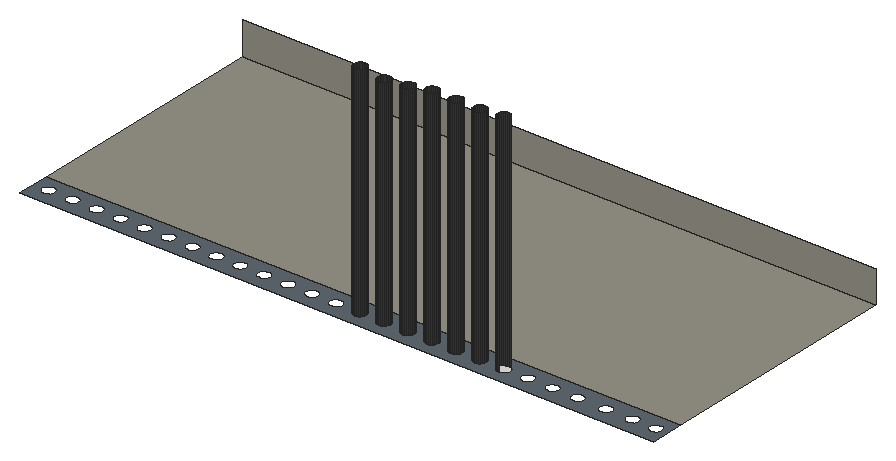
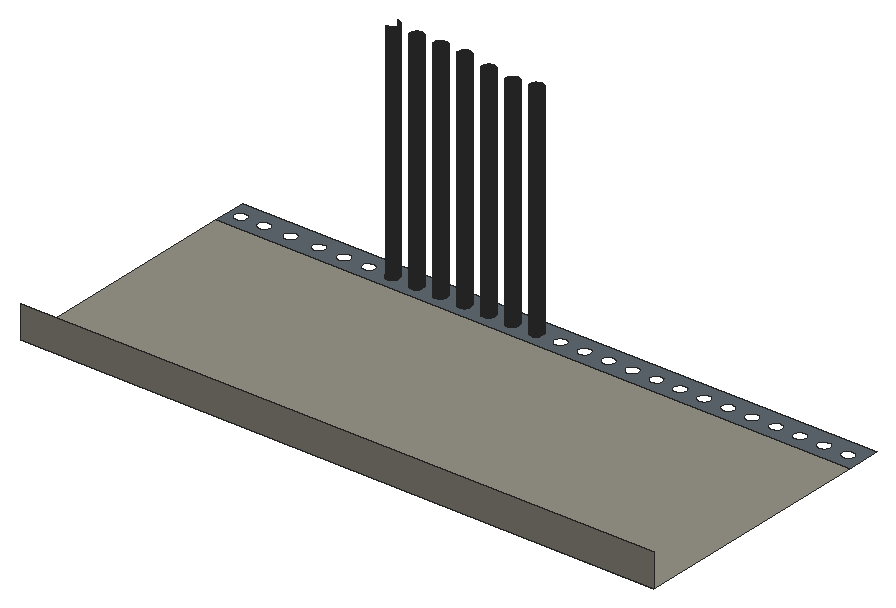
# SketchUp Ruby script. Lengths in inches.
U = 1.inch
M = Sketchup.active_model
def pt(a) = Geom::Point3d.new(a.map { |v| v * U })
def face(e, loops, mat)
  f = e.add_face(loops[0].map { |a| pt(a) })
  loops[1..].each { |l| e.add_face(l.map { |a| pt(a) }).erase! }
  f.material = f.back_material = mat if mat
  f
end
# faces: each face lists its corners as indices into pts; further lists are holes
def faces(e, pts, list, mat = nil) = list.each { |f| face(e, (f[0].is_a?(Array) ? f : [f]).map { |l| l.map { |i| pts[i] } }, mat) }
# xy, xz, yz: faces in a plane at the given z, y or x. An outline is a flat list of corners, or four numbers for a rectangle; further outlines are holes
def ring(l) = l.size == 4 ? [[l[0], l[1]], [l[2], l[1]], [l[2], l[3]], [l[0], l[3]]] : l.each_slice(2).to_a
def flat(e, list, mat, &to3) = list.each { |f| face(e, (f[0].is_a?(Array) ? f : [f]).map { |l| ring(l).map { |u, v| to3.(u, v) } }, mat) }
def xy(e, z, list, mat = nil) = flat(e, list, mat) { |x, y| [x, y, z] }
def xz(e, y, list, mat = nil) = flat(e, list, mat) { |x, z| [x, y, z] }
def yz(e, x, list, mat = nil) = flat(e, list, mat) { |y, z| [x, y, z] }
def lines(e, pts, list) = list.each { |a, b| e.add_line(pt(pts[a]), pt(pts[b])) }
# prism: a flat outline (further loops are holes) pulled along v
def prism(e, loops, v, mat = nil)
  f = face(e, loops, mat); d = Geom::Vector3d.new(v.map { |x| x * U })
  f.pushpull(f.normal.samedirection?(d) ? d.length : -d.length)
end
def box(e, o, s, mat = nil) = prism(e, [[o, [o[0] + s[0], o[1], o[2]], [o[0] + s[0], o[1] + s[1], o[2]], [o[0], o[1] + s[1], o[2]]]], [0, 0, s[2]], mat)
def at(x, y, z, deg = 0) = Geom::Transformation.translation(pt([x, y, z])) * Geom::Transformation.rotation(ORIGIN, Z_AXIS, deg.degrees)
def axes(o, x, y, z) = Geom::Transformation.new([*x, 0, *y, 0, *z, 0, *pt(o).to_a, 1])
def part(name) = M.definitions.add(name)
# library, detail: a bought-in or finely detailed component or shape, given as its bounding box
def library(name, o, s) = part(name).tap { |d| box(d.entities, o, s) }
def detail(e, o, s) = box(e.add_group.entities, o, s)
def put(e, d, t, mat = nil) = e.add_instance(d, t).tap { |i| i.material = mat if mat }
def group(e, t, mat = nil) = e.add_group.tap { |g| g.transformation = t; g.material = mat if mat }.entities
root = M.entities
M.materials.add("[Color M07]").color = [58, 58, 58]
M.materials.add("[Formica Graystone]").color = [149, 146, 135]
M.materials.add("[Formica Speckled Grey]").color = [94, 105, 111]
xy(root,557.29,[[258.98,117.55,258.8125,117.57,258.66,117.63,258.53,117.73,258.43,117.86,258.37,118.01,258.35,118.17,258.37,118.33,258.43,118.48,258.53,118.61,258.66,118.71,258.8125,118.77,258.98,118.8,259.14,118.77,259.29,118.71,259.42,118.61,259.52,118.48,259.58,118.33,259.6,118.17,259.58,118.01,259.52,117.86,259.42,117.73,259.29,117.63,259.14,117.57],[261.35,117.55,261.1875,117.57,261.04,117.63,260.91,117.73,260.81,117.86,260.75,118.01,260.73,118.17,260.75,118.33,260.81,118.48,260.91,118.61,261.04,118.71,261.1875,118.77,261.35,118.8,261.51,118.77,261.66,118.71,261.79,118.61,261.89,118.48,261.95,118.33,261.98,118.17,261.95,118.01,261.89,117.86,261.79,117.73,261.66,117.63,261.51,117.57],[263.73,117.55,263.5625,117.57,263.41,117.63,263.28,117.73,263.18,117.86,263.12,118.01,263.1,118.17,263.12,118.33,263.18,118.48,263.28,118.61,263.41,118.71,263.5625,118.77,263.73,118.8,263.89,118.77,264.04,118.71,264.17,118.61,264.27,118.48,264.33,118.33,264.35,118.17,264.33,118.01,264.27,117.86,264.17,117.73,264.04,117.63,263.89,117.57],[266.1,117.55,265.9375,117.57,265.79,117.63,265.66,117.73,265.56,117.86,265.5,118.01,265.48,118.17,265.5,118.33,265.56,118.48,265.66,118.61,265.79,118.71,265.9375,118.77,266.1,118.8,266.26,118.77,266.41,118.71,266.54,118.61,266.64,118.48,266.7,118.33,266.73,118.17,266.7,118.01,266.64,117.86,266.54,117.73,266.41,117.63,266.26,117.57],[268.48,117.55,268.3125,117.57,268.16,117.63,268.03,117.73,267.93,117.86,267.87,118.01,267.85,118.17,267.87,118.33,267.93,118.48,268.03,118.61,268.16,118.71,268.3125,118.77,268.48,118.8,268.64,118.77,268.79,118.71,268.92,118.61,269.02,118.48,269.08,118.33,269.1,118.17,269.08,118.01,269.02,117.86,268.92,117.73,268.79,117.63,268.64,117.57],
  [270.85,117.55,270.6875,117.57,270.54,117.63,270.41,117.73,270.31,117.86,270.25,118.01,270.23,118.17,270.25,118.33,270.31,118.48,270.41,118.61,270.54,118.71,270.6875,118.77,270.85,118.8,271.01,118.77,271.16,118.71,271.29,118.61,271.39,118.48,271.45,118.33,271.48,118.17,271.45,118.01,271.39,117.86,271.29,117.73,271.16,117.63,271.01,117.57],[273.23,117.55,273.0625,117.57,272.91,117.63,272.78,117.73,272.68,117.86,272.62,118.01,272.6,118.17,272.62,118.33,272.68,118.48,272.78,118.61,272.91,118.71,273.0625,118.77,273.23,118.8,273.39,118.77,273.54,118.71,273.67,118.61,273.77,118.48,273.83,118.33,273.85,118.17,273.83,118.01,273.77,117.86,273.67,117.73,273.54,117.63,273.39,117.57]])
xy(root,557.29,[[226.66,119.78,289.43,144.04]],"[Formica Graystone]")
xy(root,557.29,[[[226.66,116.47,289.43,119.78],[228.1,117.55,227.9375,117.57,227.79,117.63,227.66,117.73,227.56,117.86,227.5,118.01,227.48,118.17,227.5,118.33,227.56,118.48,227.66,118.61,227.79,118.71,227.9375,118.77,228.1,118.8,228.26,118.77,228.41,118.71,228.54,118.61,228.64,118.48,228.7,118.33,228.73,118.17,228.7,118.01,228.64,117.86,228.54,117.73,228.41,117.63,228.26,117.57],[230.48,117.55,230.3125,117.57,230.16,117.63,230.03,117.73,229.93,117.86,229.87,118.01,229.85,118.17,229.87,118.33,229.93,118.48,230.03,118.61,230.16,118.71,230.3125,118.77,230.48,118.8,230.64,118.77,230.79,118.71,230.92,118.61,231.02,118.48,231.08,118.33,231.1,118.17,231.08,118.01,231.02,117.86,230.92,117.73,230.79,117.63,230.64,117.57],[232.85,117.55,232.6875,117.57,232.54,117.63,232.41,117.73,232.31,117.86,232.25,118.01,232.23,118.17,232.25,118.33,232.31,118.48,232.41,118.61,232.54,118.71,232.6875,118.77,232.85,118.8,233.01,118.77,233.16,118.71,233.29,118.61,233.39,118.48,233.45,118.33,233.48,118.17,233.45,118.01,233.39,117.86,233.29,117.73,233.16,117.63,233.01,117.57],[235.23,117.55,235.0625,117.57,234.91,117.63,234.78,117.73,234.68,117.86,234.62,118.01,234.6,118.17,234.62,118.33,234.68,118.48,234.78,118.61,234.91,118.71,235.0625,118.77,235.23,118.8,235.39,118.77,235.54,118.71,235.67,118.61,235.77,118.48,235.83,118.33,235.85,118.17,235.83,118.01,235.77,117.86,235.67,117.73,235.54,117.63,235.39,117.57],[237.6,117.55,237.4375,117.57,237.29,117.63,237.16,117.73,237.06,117.86,237,118.01,236.98,118.17,237,118.33,237.06,118.48,237.16,118.61,237.29,118.71,237.4375,118.77,237.6,118.8,237.76,118.77,237.91,118.71,238.04,118.61,238.14,118.48,238.2,118.33,238.23,118.17,238.2,118.01,238.14,117.86,238.04,117.73,237.91,117.63,237.76,117.57],[239.98,117.55,239.8125,117.57,239.66,117.63,239.53,117.73,239.43,117.86,239.37,118.01,239.35,118.17,239.37,118.33,239.43,118.48,239.53,118.61,239.66,118.71,239.8125,118.77,239.98,118.8,240.14,118.77,240.29,118.71,240.42,118.61,240.52,118.48,240.58,118.33,240.6,118.17,240.58,118.01,240.52,117.86,240.42,117.73,240.29,117.63,240.14,117.57],[242.35,117.55,242.1875,117.57,242.04,117.63,241.91,117.73,241.81,117.86,241.75,118.01,241.73,118.17,241.75,118.33,241.81,118.48,241.91,118.61,242.04,118.71,242.1875,118.77,242.35,118.8,242.51,118.77,242.66,118.71,242.79,118.61,242.89,118.48,242.95,118.33,242.98,118.17,242.95,118.01,242.89,117.86,242.79,117.73,242.66,117.63,242.51,117.57],[244.73,117.55,244.5625,117.57,244.41,117.63,244.28,117.73,244.18,117.86,244.12,118.01,244.1,118.17,244.12,118.33,244.18,118.48,244.28,118.61,244.41,118.71,244.5625,118.77,244.73,118.8,244.89,118.77,245.04,118.71,245.17,118.61,245.27,118.48,245.33,118.33,245.35,118.17,245.33,118.01,245.27,117.86,245.17,117.73,245.04,117.63,244.89,117.57],[247.1,117.55,246.9375,117.57,246.79,117.63,246.66,117.73,246.56,117.86,246.5,118.01,246.48,118.17,246.5,118.33,246.56,118.48,246.66,118.61,246.79,118.71,246.9375,118.77,247.1,118.8,247.26,118.77,247.41,118.71,247.54,118.61,247.64,118.48,247.7,118.33,247.73,118.17,247.7,118.01,247.64,117.86,247.54,117.73,247.41,117.63,247.26,117.57],[249.48,117.55,249.3125,117.57,249.16,117.63,249.03,117.73,248.93,117.86,248.87,118.01,248.85,118.17,248.87,118.33,248.93,118.48,249.03,118.61,249.16,118.71,249.3125,118.77,249.48,118.8,249.64,118.77,249.79,118.71,249.92,118.61,250.02,118.48,250.08,118.33,250.1,118.17,250.08,118.01,250.02,117.86,249.92,117.73,249.79,117.63,249.64,117.57],[251.85,117.55,251.6875,117.57,251.54,117.63,251.41,117.73,251.31,117.86,251.25,118.01,251.23,118.17,251.25,118.33,251.31,118.48,251.41,118.61,251.54,118.71,251.6875,118.77,251.85,118.8,252.01,118.77,252.16,118.71,252.29,118.61,252.39,118.48,252.45,118.33,252.48,118.17,252.45,118.01,252.39,117.86,252.29,117.73,252.16,117.63,252.01,117.57],[254.23,117.55,254.0625,117.57,253.91,117.63,253.78,117.73,253.68,117.86,253.62,118.01,253.6,118.17,253.62,118.33,253.68,118.48,253.78,118.61,253.91,118.71,254.0625,118.77,254.23,118.8,254.39,118.77,254.54,118.71,254.67,118.61,254.77,118.48,254.83,118.33,254.85,118.17,254.83,118.01,254.77,117.86,254.67,117.73,254.54,117.63,254.39,117.57],[256.6,117.55,256.4375,117.57,256.29,117.63,256.16,117.73,256.06,117.86,256,118.01,255.98,118.17,256,118.33,256.06,118.48,256.16,118.61,256.29,118.71,256.4375,118.77,256.6,118.8,256.76,118.77,256.91,118.71,257.04,118.61,257.14,118.48,257.2,118.33,257.23,118.17,257.2,118.01,257.14,117.86,257.04,117.73,256.91,117.63,256.76,117.57],[258.98,117.55,258.8125,117.57,258.66,117.63,258.53,117.73,258.43,117.86,258.37,118.01,258.35,118.17,258.37,118.33,258.43,118.48,258.53,118.61,258.66,118.71,258.8125,118.77,258.98,118.8,259.14,118.77,259.29,118.71,259.42,118.61,259.52,118.48,259.58,118.33,259.6,118.17,259.58,118.01,259.52,117.86,259.42,117.73,259.29,117.63,259.14,117.57],[261.35,117.55,261.1875,117.57,261.04,117.63,260.91,117.73,260.81,117.86,260.75,118.01,260.73,118.17,260.75,118.33,260.81,118.48,260.91,118.61,261.04,118.71,261.1875,118.77,261.35,118.8,261.51,118.77,261.66,118.71,261.79,118.61,261.89,118.48,261.95,118.33,261.98,118.17,261.95,118.01,261.89,117.86,261.79,117.73,261.66,117.63,261.51,117.57],[263.73,117.55,263.5625,117.57,263.41,117.63,263.28,117.73,263.18,117.86,263.12,118.01,263.1,118.17,263.12,118.33,263.18,118.48,263.28,118.61,263.41,118.71,263.5625,118.77,263.73,118.8,263.89,118.77,264.04,118.71,264.17,118.61,264.27,118.48,264.33,118.33,264.35,118.17,264.33,118.01,264.27,117.86,264.17,117.73,264.04,117.63,263.89,117.57],[266.1,117.55,265.9375,117.57,265.79,117.63,265.66,117.73,265.56,117.86,265.5,118.01,265.48,118.17,265.5,118.33,265.56,118.48,265.66,118.61,265.79,118.71,265.9375,118.77,266.1,118.8,266.26,118.77,266.41,118.71,266.54,118.61,266.64,118.48,266.7,118.33,266.73,118.17,266.7,118.01,266.64,117.86,266.54,117.73,266.41,117.63,266.26,117.57],[268.48,117.55,268.3125,117.57,268.16,117.63,268.03,117.73,267.93,117.86,267.87,118.01,267.85,118.17,267.87,118.33,267.93,118.48,268.03,118.61,268.16,118.71,268.3125,118.77,268.48,118.8,268.64,118.77,268.79,118.71,268.92,118.61,269.02,118.48,269.08,118.33,269.1,118.17,269.08,118.01,269.02,117.86,268.92,117.73,268.79,117.63,268.64,117.57],[270.85,117.55,270.6875,117.57,270.54,117.63,270.41,117.73,270.31,117.86,270.25,118.01,270.23,118.17,270.25,118.33,270.31,118.48,270.41,118.61,270.54,118.71,270.6875,118.77,270.85,118.8,271.01,118.77,271.16,118.71,271.29,118.61,271.39,118.48,271.45,118.33,271.48,118.17,271.45,118.01,271.39,117.86,271.29,117.73,271.16,117.63,271.01,117.57],[273.23,117.55,273.0625,117.57,272.91,117.63,272.78,117.73,272.68,117.86,272.62,118.01,272.6,118.17,272.62,118.33,272.68,118.48,272.78,118.61,272.91,118.71,273.0625,118.77,273.23,118.8,273.39,118.77,273.54,118.71,273.67,118.61,273.77,118.48,273.83,118.33,273.85,118.17,273.83,118.01,273.77,117.86,273.67,117.73,273.54,117.63,273.39,117.57],[275.6,117.55,275.4375,117.57,275.29,117.63,275.16,117.73,275.06,117.86,275,118.01,274.98,118.17,275,118.33,275.06,118.48,275.16,118.61,275.29,118.71,275.4375,118.77,275.6,118.8,275.76,118.77,275.91,118.71,276.04,118.61,276.14,118.48,276.2,118.33,276.23,118.17,276.2,118.01,276.14,117.86,276.04,117.73,275.91,117.63,275.76,117.57],[288.29,117.55,288.125,117.57,287.98,117.63,287.85,117.73,287.75,117.86,287.68,118.01,287.66,118.17,287.68,118.33,287.75,118.48,287.85,118.61,287.98,118.71,288.125,118.77,288.29,118.8,288.45,118.77,288.6,118.71,288.73,118.61,288.83,118.48,288.89,118.33,288.91,118.17,288.89,118.01,288.83,117.86,288.73,117.73,288.6,117.63,288.45,117.57],[278.04,117.55,277.875,117.57,277.73,117.63,277.6,117.73,277.5,117.86,277.43,118.01,277.41,118.17,277.43,118.33,277.5,118.48,277.6,118.61,277.73,118.71,277.875,118.77,278.04,118.8,278.2,118.77,278.35,118.71,278.48,118.61,278.58,118.48,278.64,118.33,278.66,118.17,278.64,118.01,278.58,117.86,278.48,117.73,278.35,117.63,278.2,117.57],[285.98,117.55,285.8125,117.57,285.66,117.63,285.53,117.73,285.43,117.86,285.37,118.01,285.35,118.17,285.37,118.33,285.43,118.48,285.53,118.61,285.66,118.71,285.8125,118.77,285.98,118.8,286.14,118.77,286.29,118.71,286.42,118.61,286.52,118.48,286.58,118.33,286.6,118.17,286.58,118.01,286.52,117.86,286.42,117.73,286.29,117.63,286.14,117.57],[280.54,117.55,280.375,117.57,280.23,117.63,280.1,117.73,280,117.86,279.93,118.01,279.91,118.17,279.93,118.33,280,118.48,280.1,118.61,280.23,118.71,280.375,118.77,280.54,118.8,280.7,118.77,280.85,118.71,280.98,118.61,281.08,118.48,281.14,118.33,281.16,118.17,281.14,118.01,281.08,117.86,280.98,117.73,280.85,117.63,280.7,117.57],[283.35,117.55,283.1875,117.57,283.04,117.63,282.91,117.73,282.81,117.86,282.75,118.01,282.73,118.17,282.75,118.33,282.81,118.48,282.91,118.61,283.04,118.71,283.1875,118.77,283.35,118.8,283.51,118.77,283.66,118.71,283.79,118.61,283.89,118.48,283.95,118.33,283.98,118.17,283.95,118.01,283.89,117.86,283.79,117.73,283.66,117.63,283.51,117.57]]],"[Formica Speckled Grey]")
xz(root,144.04,[[226.66,557.29,289.43,560.54]],"[Formica Graystone]")
p = [[258.8125,117.57,557.29],[258.98,117.55,557.29],[258.98,117.55,579.17],[258.8125,117.57,579.17],[258.8125,117.57,578.7],[259.14,117.57,557.29],
  [259.14,117.57,578.7],[259.14,117.57,579.17],[261.1875,117.57,557.29],[261.35,117.55,557.29],[261.35,117.55,578.86],[261.1875,117.57,578.86],
  [261.1875,117.57,578.7],[261.51,117.57,557.29],[261.51,117.57,578.7],[261.51,117.57,578.86],[263.5625,117.57,557.29],[263.73,117.55,557.29],
  [263.73,117.55,579.11],[263.5625,117.57,579.11],[263.5625,117.57,578.7],[263.89,117.57,557.29],[263.89,117.57,578.7],[263.89,117.57,579.11],
  [265.9375,117.57,557.29],[266.1,117.55,557.29],[266.1,117.55,579.54],[265.9375,117.57,579.54],[265.9375,117.57,578.7],[266.26,117.57,557.29],
  [266.26,117.57,578.7],[266.26,117.57,579.54],[268.3125,117.57,557.29],[268.48,117.55,557.29],[268.48,117.55,579.54],[268.3125,117.57,579.54],
  [268.3125,117.57,578.7],[268.64,117.57,557.29],[268.64,117.57,578.7],[268.64,117.57,579.54],[270.6875,117.57,557.29],[270.85,117.55,557.29],
  [270.85,117.55,579.54],[270.6875,117.57,579.54],[270.6875,117.57,578.7],[271.01,117.57,557.29],[271.01,117.57,578.7],[271.01,117.57,579.54],
  [273.0625,117.57,557.29],[273.23,117.55,557.29],[273.23,117.55,579.76],[273.0625,117.57,579.76],[273.0625,117.57,578.7],[258.53,117.73,557.29],
  [258.66,117.63,557.29],[258.66,117.63,579.17],[258.53,117.73,579.17],[259.29,117.63,557.29],[259.29,117.63,579.17],[259.42,117.73,557.29],
  [259.42,117.73,579.17],[260.91,117.73,557.29],[261.04,117.63,557.29],[261.04,117.63,578.86],[260.91,117.73,578.86],[261.66,117.63,557.29],
  [261.66,117.63,578.86],[261.79,117.73,557.29],[261.79,117.73,578.86],[263.28,117.73,557.29],[263.41,117.63,557.29],[263.41,117.63,579.11],
  [263.28,117.73,579.11],[264.04,117.63,557.29],[264.04,117.63,579.11],[264.17,117.73,557.29],[264.17,117.73,579.11],[265.66,117.73,557.29],
  [265.79,117.63,557.29],[265.79,117.63,579.54],[265.66,117.73,579.54],[266.41,117.63,557.29],[266.41,117.63,579.54],[266.54,117.73,557.29],
  [266.54,117.73,579.54],[268.03,117.73,557.29],[268.16,117.63,557.29],[268.16,117.63,579.54],[268.03,117.73,579.54],[268.79,117.63,557.29],
  [268.79,117.63,579.54],[268.92,117.73,557.29],[268.92,117.73,579.54],[270.41,117.73,557.29],[270.54,117.63,557.29],[270.54,117.63,579.54],
  [270.41,117.73,579.54],[271.16,117.63,557.29],[271.16,117.63,579.54],[271.29,117.73,557.29],[271.29,117.73,579.54],[272.78,117.73,557.29],
  [272.91,117.63,557.29],[272.91,117.63,579.76],[272.78,117.73,579.76],[258.43,117.86,557.29],[258.43,117.86,579.17],[259.52,117.86,557.29],
  [259.52,117.86,579.17],[260.81,117.86,557.29],[260.81,117.86,578.86],[261.89,117.86,557.29],[261.89,117.86,578.86],[263.18,117.86,557.29],
  [263.18,117.86,579.11],[264.27,117.86,557.29],[264.27,117.86,579.11],[265.56,117.86,557.29],[265.56,117.86,579.54],[266.64,117.86,557.29],
  [266.64,117.86,579.54],[267.93,117.86,557.29],[267.93,117.86,579.54],[269.02,117.86,557.29],[269.02,117.86,579.54],[270.31,117.86,557.29],
  [270.31,117.86,579.54],[271.39,117.86,557.29],[271.39,117.86,579.54],[272.68,117.86,557.29],[272.68,117.86,579.76],[258.37,118.01,557.29],
  [258.37,118.01,579.17],[259.58,118.01,557.29],[259.58,118.01,579.17],[260.75,118.01,557.29],[260.75,118.01,578.86],[261.95,118.01,557.29],
  [261.95,118.01,578.86],[263.12,118.01,557.29],[263.12,118.01,579.11],[264.33,118.01,557.29],[264.33,118.01,579.11],[265.5,118.01,557.29],
  [265.5,118.01,579.54],[266.7,118.01,557.29],[266.7,118.01,579.54],[267.87,118.01,557.29],[267.87,118.01,579.54],[269.08,118.01,557.29],
  [269.08,118.01,579.54],[270.25,118.01,557.29],[270.25,118.01,579.54],[271.45,118.01,557.29],[271.45,118.01,579.54],[272.62,118.01,557.29],
  [272.62,118.01,579.76],[258.35,118.17,557.29],[258.35,118.17,579.17],[259.6,118.17,557.29],[259.6,118.17,579.17],[260.73,118.17,557.29],
  [260.73,118.17,578.86],[261.98,118.17,557.29],[261.98,118.17,578.86],[263.1,118.17,557.29],[263.1,118.17,579.11],[264.35,118.17,557.29],
  [264.35,118.17,579.11],[265.48,118.17,557.29],[265.48,118.17,579.54],[266.73,118.17,557.29],[266.73,118.17,579.54],[267.85,118.17,557.29],
  [267.85,118.17,579.54],[269.1,118.17,557.29],[269.1,118.17,579.54],[270.23,118.17,557.29],[270.23,118.17,579.54],[271.48,118.17,557.29],
  [271.48,118.17,579.54],[272.6,118.17,557.29],[272.6,118.17,579.76],[258.37,118.33,557.29],[258.37,118.33,579.17],[259.58,118.33,557.29],
  [259.58,118.33,579.17],[260.75,118.33,557.29],[260.75,118.33,578.86],[261.95,118.33,557.29],[261.95,118.33,578.86],[263.12,118.33,557.29],
  [263.12,118.33,579.11],[264.33,118.33,557.29],[264.33,118.33,579.11],[265.5,118.33,557.29],[265.5,118.33,579.54],[266.7,118.33,557.29],
  [266.7,118.33,579.54],[267.87,118.33,557.29],[267.87,118.33,579.54],[269.08,118.33,557.29],[269.08,118.33,579.54],[270.25,118.33,557.29],
  [270.25,118.33,579.54],[271.45,118.33,557.29],[271.45,118.33,579.54],[272.62,118.33,557.29],[272.62,118.33,579.76],[258.43,118.48,557.29],
  [258.43,118.48,579.17],[259.52,118.48,557.29],[259.52,118.48,579.17],[260.81,118.48,557.29],[260.81,118.48,578.86],[261.89,118.48,557.29],
  [261.89,118.48,578.86],[263.18,118.48,557.29],[263.18,118.48,579.11],[264.27,118.48,557.29],[264.27,118.48,579.11],[265.56,118.48,557.29],
  [265.56,118.48,579.54],[266.64,118.48,557.29],[266.64,118.48,579.54],[267.93,118.48,557.29],[267.93,118.48,579.54],[269.02,118.48,557.29],
  [269.02,118.48,579.54],[270.31,118.48,557.29],[270.31,118.48,579.54],[271.39,118.48,557.29],[271.39,118.48,579.54],[272.68,118.48,557.29],
  [272.68,118.48,579.76],[258.53,118.61,557.29],[258.53,118.61,579.17],[259.42,118.61,557.29],[259.42,118.61,579.17],[260.91,118.61,557.29],
  [260.91,118.61,578.86],[261.79,118.61,557.29],[261.79,118.61,578.86],[263.28,118.61,557.29],[263.28,118.61,579.11],[264.17,118.61,557.29],
  [264.17,118.61,579.11],[265.66,118.61,557.29],[265.66,118.61,579.54],[266.54,118.61,557.29],[266.54,118.61,579.54],[268.03,118.61,557.29],
  [268.03,118.61,579.54],[268.92,118.61,557.29],[268.92,118.61,579.54],[270.41,118.61,557.29],[270.41,118.61,579.54],[271.29,118.61,557.29],
  [271.29,118.61,579.54],[272.78,118.61,557.29],[272.78,118.61,579.76],[258.66,118.71,557.29],[258.66,118.71,579.17],[259.29,118.71,557.29],
  [259.29,118.71,579.17],[261.04,118.71,557.29],[261.04,118.71,578.86],[261.66,118.71,557.29],[261.66,118.71,578.86],[263.41,118.71,557.29],
  [263.41,118.71,579.11],[264.04,118.71,557.29],[264.04,118.71,579.11],[265.79,118.71,557.29],[265.79,118.71,579.54],[266.41,118.71,557.29],
  [266.41,118.71,579.54],[268.16,118.71,557.29],[268.16,118.71,579.54],[268.79,118.71,557.29],[268.79,118.71,579.54],[270.54,118.71,557.29],
  [270.54,118.71,579.54],[271.16,118.71,557.29],[271.16,118.71,579.54],[272.91,118.71,557.29],[272.91,118.71,579.76],[258.8125,118.77,557.29],
  [258.8125,118.77,579.17],[259.14,118.77,557.29],[259.14,118.77,579.17],[261.1875,118.77,557.29],[261.1875,118.77,578.86],[261.51,118.77,557.29],
  [261.51,118.77,578.86],[263.5625,118.77,557.29],[263.5625,118.77,579.11],[263.89,118.77,557.29],[263.89,118.77,579.11],[265.9375,118.77,557.29],
  [265.9375,118.77,579.54],[266.26,118.77,557.29],[266.26,118.77,579.54],[268.3125,118.77,557.29],[268.3125,118.77,579.54],[268.64,118.77,557.29],
  [268.64,118.77,579.54],[270.6875,118.77,557.29],[270.6875,118.77,579.54],[271.01,118.77,557.29],[271.01,118.77,579.54],[273.0625,118.77,557.29],
  [273.0625,118.77,579.76],[258.98,118.8,557.29],[258.98,118.8,579.17],[261.35,118.8,557.29],[261.35,118.8,578.86],[263.73,118.8,557.29],
  [263.73,118.8,579.11],[266.1,118.8,557.29],[266.1,118.8,579.54],[268.48,118.8,557.29],[268.48,118.8,579.54],[270.85,118.8,557.29],
  [270.85,118.8,579.54],[273.23,118.8,557.29],[273.23,118.8,579.76],[273.39,118.77,557.29],[273.39,118.77,579.76]]
faces(root,p,[[0,1,2,3,4],[1,5,6,7,2],[8,9,10,11,12],[9,13,14,15,10],[16,17,18,19,20],[17,21,22,23,18],[24,25,26,27,28],[25,29,30,31,26],
  [32,33,34,35,36],[33,37,38,39,34],[40,41,42,43,44],[41,45,46,47,42],[48,49,50,51,52],[53,54,55,56],[54,0,4,3,55],[5,57,58,7,6],
  [57,59,60,58],[61,62,63,64],[62,8,12,11,63],[13,65,66,15,14],[65,67,68,66],[69,70,71,72],[70,16,20,19,71],[21,73,74,23,22],
  [73,75,76,74],[77,78,79,80],[78,24,28,27,79],[29,81,82,31,30],[81,83,84,82],[85,86,87,88],[86,32,36,35,87],[37,89,90,39,38],
  [89,91,92,90],[93,94,95,96],[94,40,44,43,95],[45,97,98,47,46],[97,99,100,98],[101,102,103,104],[102,48,52,51,103],[105,53,56,106],
  [59,107,108,60],[109,61,64,110],[67,111,112,68],[113,69,72,114],[75,115,116,76],[117,77,80,118],[83,119,120,84],[121,85,88,122],
  [91,123,124,92],[125,93,96,126],[99,127,128,100],[129,101,104,130],[131,105,106,132],[107,133,134,108],[135,109,110,136],[111,137,138,112],
  [139,113,114,140],[115,141,142,116],[143,117,118,144],[119,145,146,120],[147,121,122,148],[123,149,150,124],[151,125,126,152],[127,153,154,128],
  [155,129,130,156],[157,131,132,158],[133,159,160,134],[161,135,136,162],[137,163,164,138],[165,139,140,166],[141,167,168,142],[169,143,144,170],
  [145,171,172,146],[173,147,148,174],[149,175,176,150],[177,151,152,178],[153,179,180,154],[181,155,156,182],[183,157,158,184],[159,185,186,160],
  [187,161,162,188],[163,189,190,164],[191,165,166,192],[167,193,194,168],[195,169,170,196],[171,197,198,172],[199,173,174,200],[175,201,202,176],
  [203,177,178,204],[179,205,206,180],[207,181,182,208],[209,183,184,210],[185,211,212,186],[213,187,188,214],[189,215,216,190],[217,191,192,218],
  [193,219,220,194],[221,195,196,222],[197,223,224,198],[225,199,200,226],[201,227,228,202],[229,203,204,230],[205,231,232,206],[233,207,208,234],
  [235,209,210,236],[211,237,238,212],[239,213,214,240],[215,241,242,216],[243,217,218,244],[219,245,246,220],[247,221,222,248],[223,249,250,224],
  [251,225,226,252],[227,253,254,228],[255,229,230,256],[231,257,258,232],[259,233,234,260],[261,235,236,262],[237,263,264,238],[265,239,240,266],
  [241,267,268,242],[269,243,244,270],[245,271,272,246],[273,247,248,274],[249,275,276,250],[277,251,252,278],[253,279,280,254],[281,255,256,282],
  [257,283,284,258],[285,259,260,286],[287,261,262,288],[263,289,290,264],[291,265,266,292],[267,293,294,268],[295,269,270,296],[271,297,298,272],
  [299,273,274,300],[275,301,302,276],[303,277,278,304],[279,305,306,280],[307,281,282,308],[283,309,310,284],[311,285,286,312],[313,287,288,314],
  [289,313,314,290],[315,291,292,316],[293,315,316,294],[317,295,296,318],[297,317,318,298],[319,299,300,320],[301,319,320,302],[321,303,304,322],
  [305,321,322,306],[323,307,308,324],[309,323,324,310],[325,311,312,326],[327,325,326,328]],"[Color M07]")
